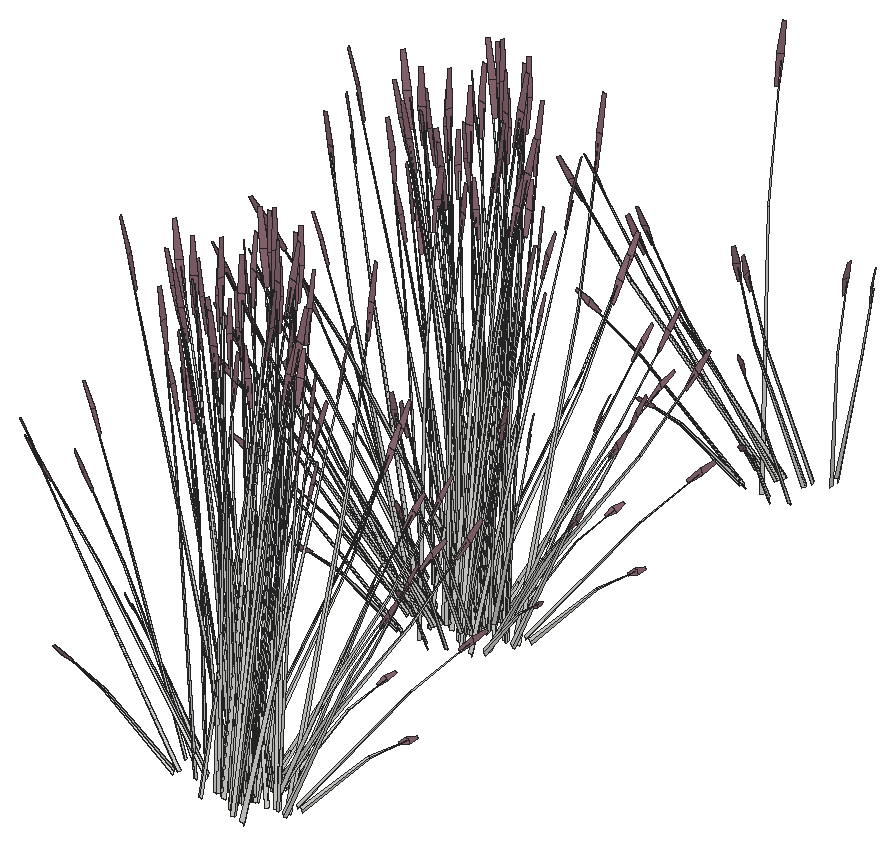
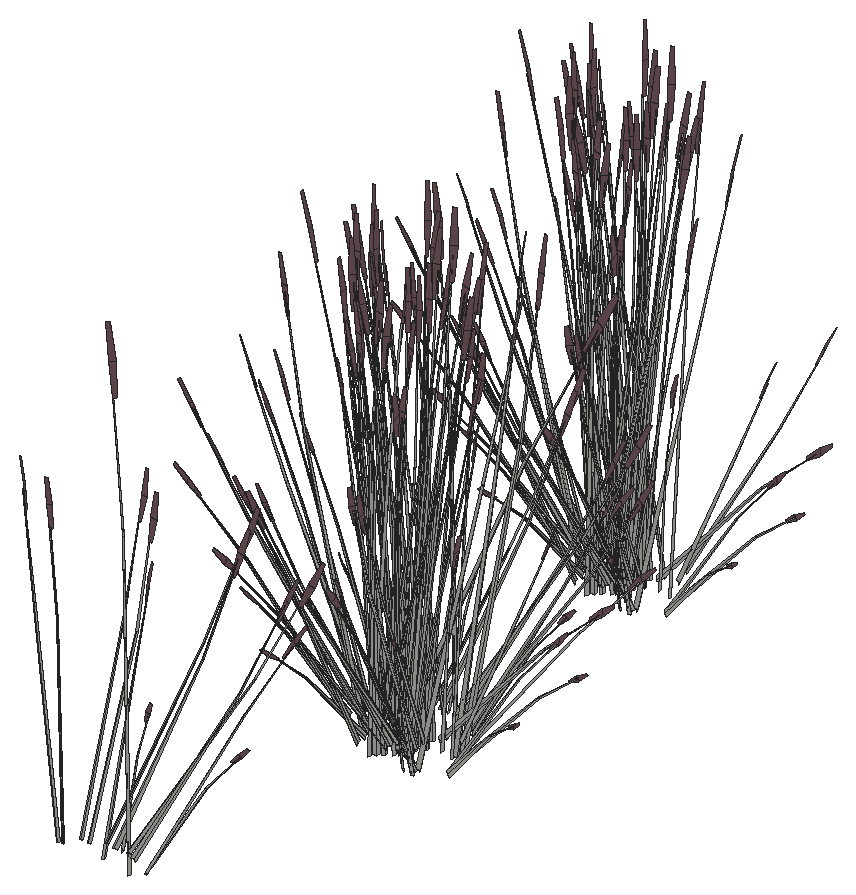
# SketchUp Ruby script. Lengths in inches.
U = 1.inch
M = Sketchup.active_model
def pt(a) = Geom::Point3d.new(a.map { |v| v * U })
def face(e, loops, mat)
  f = e.add_face(loops[0].map { |a| pt(a) })
  loops[1..].each { |l| e.add_face(l.map { |a| pt(a) }).erase! }
  f.material = f.back_material = mat if mat
  f
end
# faces: each face lists its corners as indices into pts; further lists are holes
def faces(e, pts, list, mat = nil) = list.each { |f| face(e, (f[0].is_a?(Array) ? f : [f]).map { |l| l.map { |i| pts[i] } }, mat) }
# xy, xz, yz: faces in a plane at the given z, y or x. An outline is a flat list of corners, or four numbers for a rectangle; further outlines are holes
def ring(l) = l.size == 4 ? [[l[0], l[1]], [l[2], l[1]], [l[2], l[3]], [l[0], l[3]]] : l.each_slice(2).to_a
def flat(e, list, mat, &to3) = list.each { |f| face(e, (f[0].is_a?(Array) ? f : [f]).map { |l| ring(l).map { |u, v| to3.(u, v) } }, mat) }
def xy(e, z, list, mat = nil) = flat(e, list, mat) { |x, y| [x, y, z] }
def xz(e, y, list, mat = nil) = flat(e, list, mat) { |x, z| [x, y, z] }
def yz(e, x, list, mat = nil) = flat(e, list, mat) { |y, z| [x, y, z] }
def lines(e, pts, list) = list.each { |a, b| e.add_line(pt(pts[a]), pt(pts[b])) }
# prism: a flat outline (further loops are holes) pulled along v
def prism(e, loops, v, mat = nil)
  f = face(e, loops, mat); d = Geom::Vector3d.new(v.map { |x| x * U })
  f.pushpull(f.normal.samedirection?(d) ? d.length : -d.length)
end
def box(e, o, s, mat = nil) = prism(e, [[o, [o[0] + s[0], o[1], o[2]], [o[0] + s[0], o[1] + s[1], o[2]], [o[0], o[1] + s[1], o[2]]]], [0, 0, s[2]], mat)
def at(x, y, z, deg = 0) = Geom::Transformation.translation(pt([x, y, z])) * Geom::Transformation.rotation(ORIGIN, Z_AXIS, deg.degrees)
def axes(o, x, y, z) = Geom::Transformation.new([*x, 0, *y, 0, *z, 0, *pt(o).to_a, 1])
def part(name) = M.definitions.add(name)
# library, detail: a bought-in or finely detailed component or shape, given as its bounding box
def library(name, o, s) = part(name).tap { |d| box(d.entities, o, s) }
def detail(e, o, s) = box(e.add_group.entities, o, s)
def put(e, d, t, mat = nil) = e.add_instance(d, t).tap { |i| i.material = mat if mat }
def group(e, t, mat = nil) = e.add_group.tap { |g| g.transformation = t; g.material = mat if mat }.entities
root = M.entities
M.materials.add("LightPink_Translucent").color = [144, 107, 117]
c1 = part("blade")
p = [[2.15,0.21,22],[0,0.17,0],[0.09,0.45,0],[2.18,0.31,22],[2.29,0.31,22],[0.38,0.45,0],
  [2.48,0.24,33],[2.49,0.24,33],[2.48,0.22,33]]
faces(c1.entities,p,[[0,1,2,3],[4,5,2,3],[6,3,4,7],[8,0,3,6]])
c2 = part("seeds")
p = [[0.3,-0.1,1.38],[-0.01,-0.03,1.59],[-0.01,-0.03,0.03],[0.14,-0.07,-0.07],[0.29,-0.03,3],[0.15,0.01,3.11]]
faces(c2.entities,p,[[0,1,2,3],[1,0,4,5]],"LightPink_Translucent")
c3 = part("blade with seeds")
put(c3.entities,c1,at(0,0,0))
put(c3.entities,c2,axes([2.4,0.25,30.99],[1.5799,-0.05474,1.17369],[-0.12525,1.92788,0.29478],[-0.07173,-0.02425,1.56792]))
put(root,c3,axes([48.5,471.87,44.43],[1.3808,0.50196,0.24065],[-0.66454,1.04299,0.50002],[0,-0.24043,1.60543]))
put(root,c3,axes([44.53,469.65,46.68],[-0.88986,0.68603,-0.51099],[-0.77932,-0.72471,-0.3958],[-0.45212,-0.10438,0.97773]))
put(root,c3,axes([42.53,470.5625,44.77],[0.78239,-0.07411,1.1486],[-0.49629,0.65296,0.84392],[-0.38663,-0.09795,0.25299]))
put(root,c3,axes([48.06,471.17,44.72],[-1.33077,0.06393,0.44739],[-0.12035,-1.06125,-0.21531],[0.23824,-0.10756,1.43643]))
put(root,c3,axes([44.62,471.94,44.48],[0,1.03566,0.49651],[-1.37109,0,0],[0,-0.23588,1.57504]))
put(root,c3,axes([54.25,472.17,46.68],[0.332,-0.94205,-0.51099],[1.13828,0.3229,-0.3958],[0.45829,-0.08638,0.97773]))
put(root,c3,axes([52.45,468.34,44.375],[0.7662,-1.03778,0],[1.28187,0.57875,-0.51607],[0.29196,0.13181,1.63711]))
put(root,c3,axes([48.01,471.55,44.36],[0.53281,1.15808,0.45755],[-1.52239,0.4027,0.17955],[0.01861,-0.2128,1.58856]))
put(root,c3,axes([55.46,472.4375,43.98],[-0.7893,0.12429,1.41583],[-0.12563,-0.9893,0.08104],[0.55282,-0.14974,0.80566]))
put(root,c3,axes([47.74,472.46,44.72],[-0.59459,0.93321,0.44739],[-1.23546,-0.44912,-0.21531],[0,-0.21512,1.43643]))
put(root,c3,axes([49.93,471.65,44.21],[0,-1.19833,0],[1.53239,0,0],[0,0,1.79456]))
put(root,c3,axes([51.79,468.88,44.48],[-1.14694,-0.51783,0.49651],[0.68554,-0.92854,0],[0.26122,0.11794,1.57504]))
put(root,c3,axes([54.03,472.51,46.98],[1.07686,-0.45739,-0.71045],[0.60013,0.94154,0.08574],[0.52031,-0.10696,1.00501]))
put(root,c3,axes([49.2,470.89,44.36],[-1.01611,0.93987,0.45755],[-1.20717,-0.82966,0.17955],[0.24496,-0.0938,1.58856]))
put(root,c3,axes([50.3125,472.58,44.3],[-1.1399,-0.8914,-0.06131],[1.1406,-0.89194,0],[-0.03981,-0.03113,1.75571]))
put(root,c3,axes([47.4375,469.34,44.47],[-0.35402,1.02926,0.17642],[-1.29548,-0.29127,0.35086],[0.22379,-0.00501,1.60407]))
put(root,c3,axes([50.14,470.49,44.62],[0.23642,-0.92427,0.1448],[1.15506,0.16044,-0.41347],[0.21021,0.09491,1.26744]))
put(root,c3,axes([48.14,472.68,44.36],[1.54892,0.2182,0.45755],[-0.31522,1.23236,0.17955],[-0.22636,-0.119,1.58856]))
put(root,c3,axes([49.65,470.73,44.72],[-0.73619,-0.86927,0.44739],[1.11511,-0.61213,-0.21531],[0.23824,0.10756,1.43643]))
put(root,c3,axes([47.3125,474.65,44.47],[1.31687,-0.27488,0.17642],[0.32517,1.02297,0.35086],[-0.11745,-0.14905,1.60407]))
put(root,c3,axes([50.97,471.91,44.21],[1.37109,0,0],[0,1.07219,0],[0,0,1.78407]))
put(root,c3,axes([51.36,469.4,44.47],[-1.31687,0.27488,0.17642],[-0.32517,-1.02297,0.35086],[0.11745,0.14905,1.60407]))
put(root,c3,axes([50.52,471.37,44.38],[-1.54892,-0.2182,0.49198],[0.31522,-1.23236,0.19306],[0.22636,0.119,1.70813]))
put(root,c3,axes([49.29,474.41,44.2],[-0.39985,-0.89288,0],[1.1418,-0.31268,0],[0,0,1.54371]))
put(root,c3,axes([48.53,473.56,44.62],[-0.23642,0.92427,0.1448],[-1.15506,-0.16044,-0.41347],[-0.21021,-0.09491,1.26744]))
put(root,c3,axes([51.23,474.71,44.47],[0.35402,-1.02926,0.17642],[1.29548,0.29127,0.35086],[-0.22379,0.00501,1.60407]))
put(root,c3,axes([50.9375,472.375,44.21],[0.85545,0.66896,0],[-0.85545,0.66896,0],[0,0,1.69266]))
put(root,c3,axes([46.07,471.12,45.34],[0.34834,-0.14982,1.77064],[0.12012,1.04605,0.13857],[-0.75452,0.1388,0.63284]))
put(root,c3,axes([53.25,472.08,44.47],[-0.96285,-0.75439,0.17642],[0.97031,-0.7317,0.35086],[-0.10634,0.15406,1.60407]))
put(root,c3,axes([57.1,472.77,44.77],[-0.75718,0.17097,1.1486],[0.35641,-0.70661,0.84392],[0.40168,0.04835,0.25299]))
put(root,c3,axes([49.01,474.82,44.2],[-1.23546,-0.46496,0],[0.59459,-0.96613,0],[0,0,1.62707]))
put(root,c3,axes([46.88,475.18,44.48],[1.14694,0.51783,0.49651],[-0.68554,0.92854,0],[-0.26122,-0.11794,1.57504]))
put(root,c3,axes([50.93,471.59,44.72],[0.59459,-0.93321,0.44739],[1.23546,0.44912,-0.21531],[0,0.21512,1.43643]))
put(root,c3,axes([50.7,472.125,44.29],[0,1.19774,-0.05637],[-1.53239,0,0],[0,0.03764,1.79368]))
put(root,c3,axes([43.67,471.6875,46.68],[-0.332,0.94205,-0.51099],[-1.13828,-0.3229,-0.3958],[-0.45829,0.08638,0.97773]))
put(root,c3,axes([46.22,475.72,44.375],[-0.7662,1.03778,0],[-1.28187,-0.57875,-0.51607],[-0.29196,-0.13181,1.63711]))
put(root,c3,axes([54.05,472.11,44.48],[0,-1.03566,0.49651],[1.37109,0,0],[0,0.23588,1.57504]))
put(root,c3,axes([50.61,472.89,44.72],[1.33077,-0.06393,0.44739],[0.12035,1.06125,-0.21531],[-0.23824,0.10756,1.43643]))
put(root,c3,axes([51.44,471.8,44.62],[1.1418,-0.30203,0.1448],[0.39985,0.86246,-0.41347],[0,0.18981,1.26744]))
put(root,c3,axes([55.69,473.91,44.59],[-0.29514,-0.25472,1.43002],[0.38401,-0.84262,-0.30754],[0.59714,0.11414,0.61141]))
put(root,c3,axes([50.41,474.83,44.2],[1.23546,0.46496,0],[-0.59459,0.96613,0],[0,0,1.74954]))
put(root,c3,axes([50.9,475.86,44.19],[-0.75665,-1.04141,-0.05142],[1.28187,-0.57875,0.51607],[-0.31588,0.09915,1.6363]))
put(root,c3,axes([50.63,473.34,44.62],[0.90538,0.62224,0.1448],[-0.75521,0.70202,-0.41347],[-0.21021,0.09491,1.26744]))
put(root,c3,axes([52.98,474.42,46.98],[1.22504,0.02494,-0.71045],[-0.08228,1.05005,0.08574],[0.51899,0.11081,1.00501]))
put(root,c3,axes([51.6,475.26,44.48],[1.14694,-0.51783,0.49651],[0.68554,0.92854,0],[-0.26122,0.11794,1.57504]))
put(root,c3,axes([49.97,474.44,44.29],[0.53281,1.18979,-0.06012],[-1.52239,0.41691,0],[0.01861,0.04155,1.72173]))
put(root,c3,axes([42.31,473.9,44.59],[0.42589,0.08502,1.43002],[0.2745,0.86839,-0.30754],[-0.57851,0.16255,0.61141]))
put(root,c3,axes([54.98,472.29,44.375],[1.53239,0,0],[0,1.1575,-0.51607],[0,0.26363,1.63711]))
put(root,c3,axes([54.37,472.88,44.2],[-1.53164,-0.00828,-0.04976],[0,-1.1575,0.49943],[-0.04813,0.2635,1.58352]))
put(root,c3,axes([41.42,475.72,44.77],[0.51072,-0.46938,1.1486],[0.20153,0.74307,0.84392],[-0.36908,0.13305,0.25299]))
put(root,c3,axes([50.94,475.33,44.33],[1.53422,0.33662,0.30756],[-0.38383,1.20322,-0.36492],[-0.25393,0.15059,1.64885]))
put(root,c3,axes([52.89,475.22,44.77],[-0.69001,-0.29779,1.1486],[0.89096,-0.30257,0.84392],[0.24031,0.2563,0.25299]))
put(root,c3,axes([44.23,473.79,46.68],[0.31482,0.94565,-0.51099],[-1.19224,0.16542,-0.3958],[-0.34166,0.254,0.97773]))
put(root,c3,axes([51.87,475.98,44.375],[0.7662,1.03778,0],[-1.28187,0.57875,-0.51607],[-0.29196,0.13181,1.63711]))
put(root,c3,axes([51.21,471.87,44.84],[-0.03348,-0.97511,1.41272],[1.51511,0.25277,0.59816],[-0.35835,0.53357,1.3335]))
put(root,c3,axes([51.33,475.63,46.68],[1.20928,-0.24619,-0.51099],[0.21154,0.93233,-0.3958],[0.32481,0.26718,0.97773]))
put(root,c3,axes([53,476.58,44.67],[-0.78586,-0.03248,1.0506],[0.51898,-0.68985,0.58006],[0.31045,0.24509,0.8241]))
put(root,c3,axes([50.4375,474.9,44.59],[0.02163,-0.34331,1.43002],[1.03345,-0.38348,-0.30754],[0.31903,0.4109,0.61141]))
put(root,c3,axes([45.75,477.77,44.77],[-0.03171,-0.6158,1.1486],[0.7925,0.43922,0.84392],[-0.15586,0.29352,0.25299]))
put(root,c3,axes([46.05,475.39,47],[0.87728,0.69587,-0.5672],[-0.92674,0.60943,-0.43934],[-0.13348,0.35356,1.08528]))
put(root,c3,axes([45.1,476.44,44.82],[1.11329,-0.1834,0.06507],[0.25594,0.73887,-0.86304],[-0.07058,0.37403,0.7736]))
put(root,c3,axes([48.65,476.06,46.68],[1.20468,0.25962,-0.51099],[-0.41292,0.89013,-0.3958],[0.11046,0.35838,0.97773]))
put(root,c3,axes([45.78,475.07,47.34],[-0.03189,0.95798,-0.7886],[-1.34277,-0.06434,0.09517],[-0.14171,0.40585,1.11556]))
put(root,c3,axes([48.21,475.9,46.98],[0.5849,0.8421,-0.71045],[-1.20401,0.4693,0.08574],[0.13677,0.40688,1.00501]))
put(root,c3,axes([44.83,477.22,44.59],[0.38672,-0.16338,1.43002],[0.95481,0.49262,-0.30754],[-0.28419,0.42626,0.61141]))
put(root,c3,axes([45.33,476.42,45.36],[0.02693,-0.53464,1.54345],[1.21102,0.2824,0.21329],[-0.10493,0.5698,0.72882]))
put(root,c3,axes([47.68,507.49,44.59],[-0.34835,0.20963,1.43002],[-1.04325,-0.36691,-0.30754],[0.19338,-0.4563,0.61141]))
put(root,c3,axes([46.09,508.22,46.98],[-0.5849,-0.8421,-0.71045],[1.20401,-0.4693,0.08574],[-0.13677,-0.40688,1.00501]))
put(root,c3,axes([42.29,507.1,44.59],[-0.07421,0.33879,1.43002],[-1.08488,0.28361,-0.30754],[-0.25359,-0.4379,0.61141]))
put(root,c3,axes([48.53,509.05,46.98],[0.03189,-0.95798,-0.71045],[1.34277,0.06434,0.08574],[0.14171,-0.40585,1.00501]))
put(root,c3,axes([45.65,508.05,46.68],[-1.20468,-0.25962,-0.51099],[0.41292,-0.89013,-0.3958],[-0.11046,-0.35838,0.97773]))
put(root,c3,axes([46.4,505.82,44.77],[0.15721,0.60392,1.1486],[-0.87211,-0.33448,0.84392],[0.09385,-0.30923,0.25299]))
put(root,c3,axes([48.25,508.73,46.68],[-0.87728,-0.69587,-0.51099],[0.92674,-0.60943,-0.3958],[0.13348,-0.35356,0.97773]))
put(root,c3,axes([41.91,506.55,44.77],[0.63926,0.36046,1.1486],[-0.93099,0.21668,0.84392],[-0.1992,-0.27702,0.25299]))
put(root,c3,axes([43.46,508.46,46.98],[-1.04497,-0.50058,-0.71045],[0.74264,-0.8772,0.08574],[-0.3786,-0.29889,1.00501]))
put(root,c3,axes([42.97,508.49,46.68],[-1.20928,0.24619,-0.51099],[-0.21154,-0.93233,-0.3958],[-0.32481,-0.26718,0.97773]))
put(root,c3,axes([50.11,510.71,46.98],[0.64013,-0.81717,-0.71045],[1.12174,0.58074,0.08574],[0.38221,-0.29607,1.00501]))
put(root,c3,axes([43.1875,508.33,44.375],[-0.7662,-1.03778,0],[1.28187,-0.57875,-0.51607],[0.29196,-0.13181,1.63711]))
put(root,c3,axes([50.08,510.33,46.68],[-0.31482,-0.94565,-0.51099],[1.19224,-0.16542,-0.3958],[0.34166,-0.254,0.97773]))
put(root,c3,axes([45.96,514.125,45.33],[1.05902,0.41762,1.51261],[-1.03748,0.89969,0.59816],[-0.46471,-0.53324,1.26806]))
put(root,c3,axes([51.04,509.96,44.59],[-0.4378,-0.03068,1.43002],[-0.44851,-0.8229,-0.30754],[0.53783,-0.23279,0.61141]))
put(root,c3,axes([51.54,508.45,44.77],[-0.40819,0.5272,1.1486],[-0.35086,-0.70831,0.84392],[0.33713,-0.17749,0.25299]))
put(root,c3,axes([40.08,512.02,44.375],[-1.53239,0,0],[0,-1.1575,-0.51607],[0,-0.26363,1.63711]))
put(root,c3,axes([40.34,509.95,44.59],[0.23927,0.28834,1.43002],[-0.55135,0.78376,-0.30754],[-0.56612,-0.18733,0.61141]))
put(root,c3,axes([41.33,509.7,46.98],[-1.22504,-0.02494,-0.71045],[0.08228,-1.05005,0.08574],[-0.51899,-0.11081,1.00501]))
put(root,c3,axes([41.26,511.72,44.33],[-1.1399,0.87071,0.30756],[-1.1406,-0.86155,-0.36492],[-0.03981,-0.24727,1.64885]))
put(root,c3,axes([44.89,512.125,44.43],[1.3808,0.50196,0.24065],[-0.66454,1.04299,0.50002],[0,-0.24043,1.60543]))
put(root,c3,axes([40.92,509.91,46.68],[-0.88986,0.68603,-0.51099],[-0.77932,-0.72471,-0.3958],[-0.45212,-0.10438,0.97773]))
put(root,c3,axes([38.91,510.82,44.77],[0.78239,-0.07411,1.1486],[-0.49629,0.65296,0.84392],[-0.38663,-0.09795,0.25299]))
put(root,c3,axes([44.44,511.42,44.72],[-1.33077,0.06393,0.44739],[-0.12035,-1.06125,-0.21531],[0.23824,-0.10756,1.43643]))
put(root,c3,axes([41.01,512.2,44.48],[0,1.03566,0.49651],[-1.37109,0,0],[0,-0.23588,1.57504]))
put(root,c3,axes([50.63,512.43,46.68],[0.332,-0.94205,-0.51099],[1.13828,0.3229,-0.3958],[0.45829,-0.08638,0.97773]))
put(root,c3,axes([48.83,508.59,44.375],[0.7662,-1.03778,0],[1.28187,0.57875,-0.51607],[0.29196,0.13181,1.63711]))
put(root,c3,axes([44.4,511.81,44.36],[0.53281,1.15808,0.45755],[-1.52239,0.4027,0.17955],[0.01861,-0.2128,1.58856]))
put(root,c3,axes([51.85,512.7,43.98],[-0.7893,0.12429,1.41583],[-0.12563,-0.9893,0.08104],[0.55282,-0.14974,0.80566]))
put(root,c3,axes([44.13,512.72,44.72],[-0.59459,0.93321,0.44739],[-1.23546,-0.44912,-0.21531],[0,-0.21512,1.43643]))
put(root,c3,axes([46.3125,511.91,44.21],[0,-1.19833,0],[1.53239,0,0],[0,0,1.79456]))
put(root,c3,axes([48.17,509.14,44.48],[-1.14694,-0.51783,0.49651],[0.68554,-0.92854,0],[0.26122,0.11794,1.57504]))
put(root,c3,axes([50.41,512.77,46.98],[1.07686,-0.45739,-0.71045],[0.60013,0.94154,0.08574],[0.52031,-0.10696,1.00501]))
put(root,c3,axes([45.59,511.15,44.36],[-1.01611,0.93987,0.45755],[-1.20717,-0.82966,0.17955],[0.24496,-0.0938,1.58856]))
put(root,c3,axes([46.7,512.83,44.3],[-1.1399,-0.8914,-0.06131],[1.1406,-0.89194,0],[-0.03981,-0.03113,1.75571]))
put(root,c3,axes([43.82,509.6,44.47],[-0.35402,1.02926,0.17642],[-1.29548,-0.29127,0.35086],[0.22379,-0.00501,1.60407]))
put(root,c3,axes([46.53,510.75,44.62],[0.23642,-0.92427,0.1448],[1.15506,0.16044,-0.41347],[0.21021,0.09491,1.26744]))
put(root,c3,axes([44.53,512.94,44.36],[1.54892,0.2182,0.45755],[-0.31522,1.23236,0.17955],[-0.22636,-0.119,1.58856]))
put(root,c3,axes([46.03,510.99,44.72],[-0.73619,-0.86927,0.44739],[1.11511,-0.61213,-0.21531],[0.23824,0.10756,1.43643]))
put(root,c3,axes([43.7,514.91,44.47],[1.31687,-0.27488,0.17642],[0.32517,1.02297,0.35086],[-0.11745,-0.14905,1.60407]))
put(root,c3,axes([47.35,512.17,44.21],[1.37109,0,0],[0,1.07219,0],[0,0,1.78407]))
put(root,c3,axes([47.74,509.66,44.47],[-1.31687,0.27488,0.17642],[-0.32517,-1.02297,0.35086],[0.11745,0.14905,1.60407]))
put(root,c3,axes([46.91,511.63,44.38],[-1.54892,-0.2182,0.49198],[0.31522,-1.23236,0.19306],[0.22636,0.119,1.70813]))
put(root,c3,axes([45.68,514.67,44.2],[-0.39985,-0.89288,0],[1.1418,-0.31268,0],[0,0,1.54371]))
put(root,c3,axes([44.91,513.82,44.62],[-0.23642,0.92427,0.1448],[-1.15506,-0.16044,-0.41347],[-0.21021,-0.09491,1.26744]))
put(root,c3,axes([47.62,514.97,44.47],[0.35402,-1.02926,0.17642],[1.29548,0.29127,0.35086],[-0.22379,0.00501,1.60407]))
put(root,c3,axes([47.32,512.63,44.21],[0.85545,0.66896,0],[-0.85545,0.66896,0],[0,0,1.69266]))
put(root,c3,axes([42.46,511.375,45.34],[0.34834,-0.14982,1.77064],[0.12012,1.04605,0.13857],[-0.75452,0.1388,0.63284]))
put(root,c3,axes([49.64,512.34,44.47],[-0.96285,-0.75439,0.17642],[0.97031,-0.7317,0.35086],[-0.10634,0.15406,1.60407]))
put(root,c3,axes([53.49,513.03,44.77],[-0.75718,0.17097,1.1486],[0.35641,-0.70661,0.84392],[0.40168,0.04835,0.25299]))
put(root,c3,axes([45.39,515.07,44.2],[-1.23546,-0.46496,0],[0.59459,-0.96613,0],[0,0,1.62707]))
put(root,c3,axes([43.27,515.43,44.48],[1.14694,0.51783,0.49651],[-0.68554,0.92854,0],[-0.26122,-0.11794,1.57504]))
put(root,c3,axes([47.3125,511.85,44.72],[0.59459,-0.93321,0.44739],[1.23546,0.44912,-0.21531],[0,0.21512,1.43643]))
put(root,c3,axes([47.08,512.38,44.29],[0,1.19774,-0.05637],[-1.53239,0,0],[0,0.03764,1.79368]))
put(root,c3,axes([40.06,511.95,46.68],[-0.332,0.94205,-0.51099],[-1.13828,-0.3229,-0.3958],[-0.45829,0.08638,0.97773]))
put(root,c3,axes([42.61,515.98,44.375],[-0.7662,1.03778,0],[-1.28187,-0.57875,-0.51607],[-0.29196,-0.13181,1.63711]))
put(root,c3,axes([50.43,512.37,44.48],[0,-1.03566,0.49651],[1.37109,0,0],[0,0.23588,1.57504]))
put(root,c3,axes([47,513.14,44.72],[1.33077,-0.06393,0.44739],[0.12035,1.06125,-0.21531],[-0.23824,0.10756,1.43643]))
put(root,c3,axes([47.83,512.0625,44.62],[1.1418,-0.30203,0.1448],[0.39985,0.86246,-0.41347],[0,0.18981,1.26744]))
put(root,c3,axes([52.07,514.16,44.59],[-0.29514,-0.25472,1.43002],[0.38401,-0.84262,-0.30754],[0.59714,0.11414,0.61141]))
put(root,c3,axes([46.79,515.09,44.2],[1.23546,0.46496,0],[-0.59459,0.96613,0],[0,0,1.74954]))
put(root,c3,axes([47.29,516.12,44.19],[-0.75665,-1.04141,-0.05142],[1.28187,-0.57875,0.51607],[-0.31588,0.09915,1.6363]))
put(root,c3,axes([47.02,513.6,44.62],[0.90538,0.62224,0.1448],[-0.75521,0.70202,-0.41347],[-0.21021,0.09491,1.26744]))
put(root,c3,axes([49.36,514.68,46.98],[1.22504,0.02494,-0.71045],[-0.08228,1.05005,0.08574],[0.51899,0.11081,1.00501]))
put(root,c3,axes([47.98,515.52,44.48],[1.14694,-0.51783,0.49651],[0.68554,0.92854,0],[-0.26122,0.11794,1.57504]))
put(root,c3,axes([46.35,514.7,44.29],[0.53281,1.18979,-0.06012],[-1.52239,0.41691,0],[0.01861,0.04155,1.72173]))
put(root,c3,axes([38.69,514.16,44.59],[0.42589,0.08502,1.43002],[0.2745,0.86839,-0.30754],[-0.57851,0.16255,0.61141]))
put(root,c3,axes([51.36,512.55,44.375],[1.53239,0,0],[0,1.1575,-0.51607],[0,0.26363,1.63711]))
put(root,c3,axes([50.75,513.14,44.2],[-1.53164,-0.00828,-0.04976],[0,-1.1575,0.49943],[-0.04813,0.2635,1.58352]))
put(root,c3,axes([37.8,515.98,44.77],[0.51072,-0.46938,1.1486],[0.20153,0.74307,0.84392],[-0.36908,0.13305,0.25299]))
put(root,c3,axes([47.32,515.59,44.33],[1.53422,0.33662,0.30756],[-0.38383,1.20322,-0.36492],[-0.25393,0.15059,1.64885]))
put(root,c3,axes([49.28,515.48,44.77],[-0.69001,-0.29779,1.1486],[0.89096,-0.30257,0.84392],[0.24031,0.2563,0.25299]))
put(root,c3,axes([40.61,514.05,46.68],[0.31482,0.94565,-0.51099],[-1.19224,0.16542,-0.3958],[-0.34166,0.254,0.97773]))
put(root,c3,axes([48.25,516.24,44.375],[0.7662,1.03778,0],[-1.28187,0.57875,-0.51607],[-0.29196,0.13181,1.63711]))
put(root,c3,axes([47.6,512.13,44.84],[-0.03348,-0.97511,1.41272],[1.51511,0.25277,0.59816],[-0.35835,0.53357,1.3335]))
put(root,c3,axes([47.72,515.89,46.68],[1.20928,-0.24619,-0.51099],[0.21154,0.93233,-0.3958],[0.32481,0.26718,0.97773]))
put(root,c3,axes([49.39,516.84,44.67],[-0.78586,-0.03248,1.0506],[0.51898,-0.68985,0.58006],[0.31045,0.24509,0.8241]))
put(root,c3,axes([46.82,515.16,44.59],[0.02163,-0.34331,1.43002],[1.03345,-0.38348,-0.30754],[0.31903,0.4109,0.61141]))
put(root,c3,axes([42.14,518.02,44.77],[-0.03171,-0.6158,1.1486],[0.7925,0.43922,0.84392],[-0.15586,0.29352,0.25299]))
put(root,c3,axes([42.43,515.65,47],[0.87728,0.69587,-0.5672],[-0.92674,0.60943,-0.43934],[-0.13348,0.35356,1.08528]))
put(root,c3,axes([41.48,516.69,44.82],[1.11329,-0.1834,0.06507],[0.25594,0.73887,-0.86304],[-0.07058,0.37403,0.7736]))
put(root,c3,axes([45.03,516.32,46.68],[1.20468,0.25962,-0.51099],[-0.41292,0.89013,-0.3958],[0.11046,0.35838,0.97773]))
put(root,c3,axes([42.16,515.33,47.34],[-0.03189,0.95798,-0.7886],[-1.34277,-0.06434,0.09517],[-0.14171,0.40585,1.11556]))
put(root,c3,axes([44.6,516.15,46.98],[0.5849,0.8421,-0.71045],[-1.20401,0.4693,0.08574],[0.13677,0.40688,1.00501]))
put(root,c3,axes([41.21,517.48,44.59],[0.38672,-0.16338,1.43002],[0.95481,0.49262,-0.30754],[-0.28419,0.42626,0.61141]))
put(root,c3,axes([41.71,516.68,45.36],[0.02693,-0.53464,1.54345],[1.21102,0.2824,0.21329],[-0.10493,0.5698,0.72882]))
put(root,c3,axes([55.65,551.17,44.59],[-0.34835,0.20963,1.43002],[-1.04325,-0.36691,-0.30754],[0.19338,-0.4563,0.61141]))
put(root,c3,axes([54.06,551.9,46.98],[-0.5849,-0.8421,-0.71045],[1.20401,-0.4693,0.08574],[-0.13677,-0.40688,1.00501]))
put(root,c3,axes([50.25,550.77,44.59],[-0.07421,0.33879,1.43002],[-1.08488,0.28361,-0.30754],[-0.25359,-0.4379,0.61141]))
put(root,c3,axes([56.49,552.72,46.98],[0.03189,-0.95798,-0.71045],[1.34277,0.06434,0.08574],[0.14171,-0.40585,1.00501]))
put(root,c3,axes([53.62,551.73,46.68],[-1.20468,-0.25962,-0.51099],[0.41292,-0.89013,-0.3958],[-0.11046,-0.35838,0.97773]))
put(root,c3,axes([54.37,549.5,44.77],[0.15721,0.60392,1.1486],[-0.87211,-0.33448,0.84392],[0.09385,-0.30923,0.25299]))
put(root,c3,axes([56.22,552.4,46.68],[-0.87728,-0.69587,-0.51099],[0.92674,-0.60943,-0.3958],[0.13348,-0.35356,0.97773]))
put(root,c3,axes([49.88,550.23,44.77],[0.63926,0.36046,1.1486],[-0.93099,0.21668,0.84392],[-0.1992,-0.27702,0.25299]))
put(root,c3,axes([51.42,552.14,46.98],[-1.04497,-0.50058,-0.71045],[0.74264,-0.8772,0.08574],[-0.3786,-0.29889,1.00501]))
put(root,c3,axes([50.94,552.16,46.68],[-1.20928,0.24619,-0.51099],[-0.21154,-0.93233,-0.3958],[-0.32481,-0.26718,0.97773]))
put(root,c3,axes([58.08,554.39,46.98],[0.64013,-0.81717,-0.71045],[1.12174,0.58074,0.08574],[0.38221,-0.29607,1.00501]))
put(root,c3,axes([51.16,552.01,44.375],[-0.7662,-1.03778,0],[1.28187,-0.57875,-0.51607],[0.29196,-0.13181,1.63711]))
put(root,c3,axes([58.05,554.01,46.68],[-0.31482,-0.94565,-0.51099],[1.19224,-0.16542,-0.3958],[0.34166,-0.254,0.97773]))
